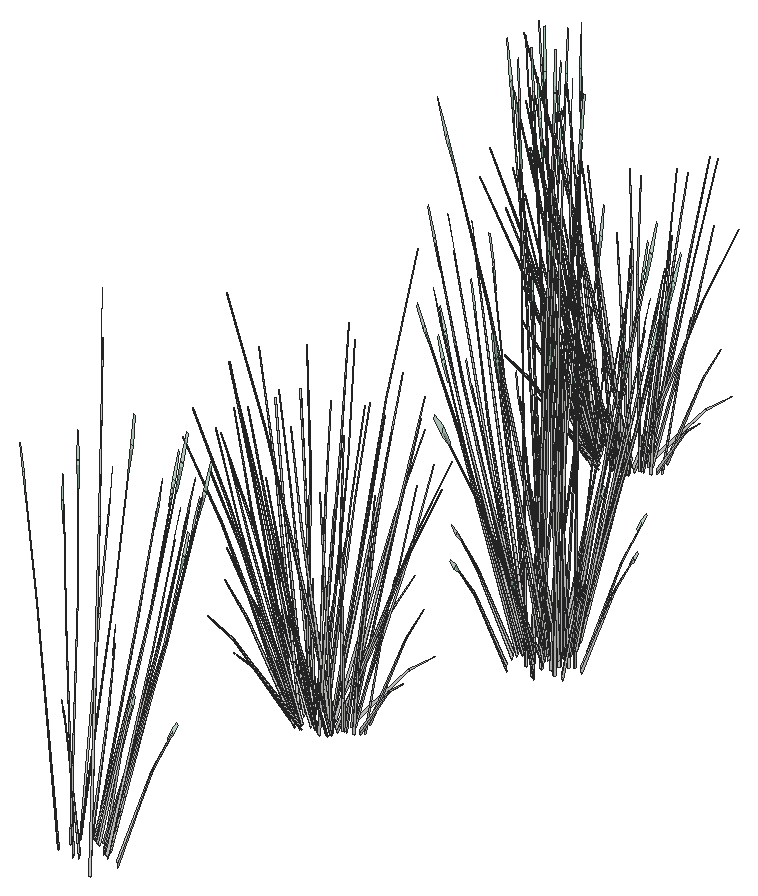
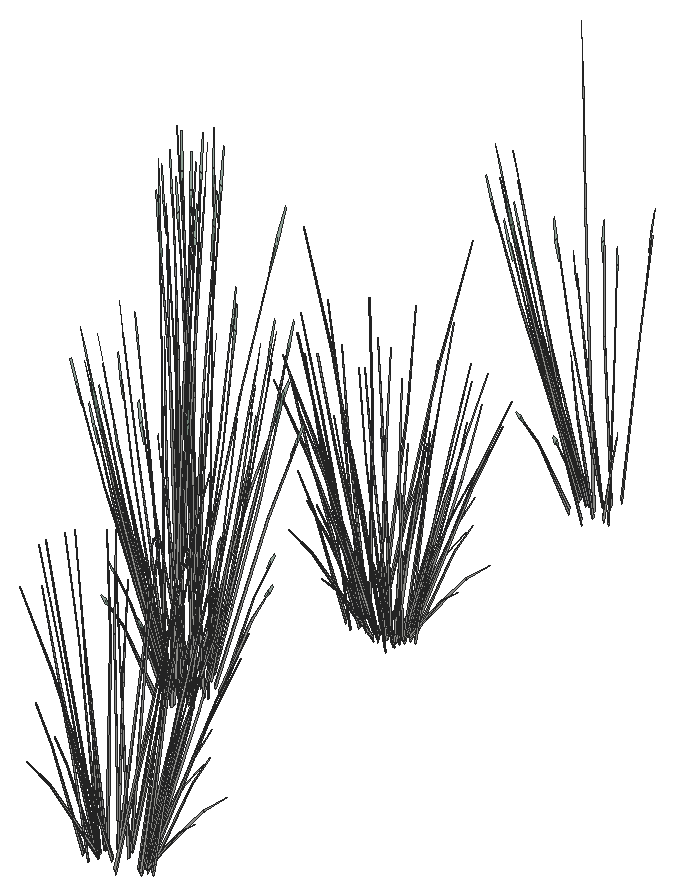
# SketchUp Ruby script. Lengths in inches.
U = 1.inch
M = Sketchup.active_model
def pt(a) = Geom::Point3d.new(a.map { |v| v * U })
def face(e, loops, mat)
  f = e.add_face(loops[0].map { |a| pt(a) })
  loops[1..].each { |l| e.add_face(l.map { |a| pt(a) }).erase! }
  f.material = f.back_material = mat if mat
  f
end
# faces: each face lists its corners as indices into pts; further lists are holes
def faces(e, pts, list, mat = nil) = list.each { |f| face(e, (f[0].is_a?(Array) ? f : [f]).map { |l| l.map { |i| pts[i] } }, mat) }
# xy, xz, yz: faces in a plane at the given z, y or x. An outline is a flat list of corners, or four numbers for a rectangle; further outlines are holes
def ring(l) = l.size == 4 ? [[l[0], l[1]], [l[2], l[1]], [l[2], l[3]], [l[0], l[3]]] : l.each_slice(2).to_a
def flat(e, list, mat, &to3) = list.each { |f| face(e, (f[0].is_a?(Array) ? f : [f]).map { |l| ring(l).map { |u, v| to3.(u, v) } }, mat) }
def xy(e, z, list, mat = nil) = flat(e, list, mat) { |x, y| [x, y, z] }
def xz(e, y, list, mat = nil) = flat(e, list, mat) { |x, z| [x, y, z] }
def yz(e, x, list, mat = nil) = flat(e, list, mat) { |y, z| [x, y, z] }
def lines(e, pts, list) = list.each { |a, b| e.add_line(pt(pts[a]), pt(pts[b])) }
# prism: a flat outline (further loops are holes) pulled along v
def prism(e, loops, v, mat = nil)
  f = face(e, loops, mat); d = Geom::Vector3d.new(v.map { |x| x * U })
  f.pushpull(f.normal.samedirection?(d) ? d.length : -d.length)
end
def box(e, o, s, mat = nil) = prism(e, [[o, [o[0] + s[0], o[1], o[2]], [o[0] + s[0], o[1] + s[1], o[2]], [o[0], o[1] + s[1], o[2]]]], [0, 0, s[2]], mat)
def at(x, y, z, deg = 0) = Geom::Transformation.translation(pt([x, y, z])) * Geom::Transformation.rotation(ORIGIN, Z_AXIS, deg.degrees)
def axes(o, x, y, z) = Geom::Transformation.new([*x, 0, *y, 0, *z, 0, *pt(o).to_a, 1])
def part(name) = M.definitions.add(name)
# library, detail: a bought-in or finely detailed component or shape, given as its bounding box
def library(name, o, s) = part(name).tap { |d| box(d.entities, o, s) }
def detail(e, o, s) = box(e.add_group.entities, o, s)
def put(e, d, t, mat = nil) = e.add_instance(d, t).tap { |i| i.material = mat if mat }
def group(e, t, mat = nil) = e.add_group.tap { |g| g.transformation = t; g.material = mat if mat }.entities
root = M.entities
M.materials.add("LightPink_Translucent").color = [175, 214, 192]
M.materials["LightPink_Translucent"].alpha = 0.75
c1 = part("blade")
p = [[2.15,0.21,22],[0,0.17,0],[0.09,0.45,0],[2.18,0.31,22],[2.29,0.31,22],[0.38,0.45,0],
  [2.48,0.24,33],[2.49,0.24,33],[2.48,0.22,33]]
faces(c1.entities,p,[[0,1,2,3],[4,5,2,3],[6,3,4,7],[8,0,3,6]])
c2 = part("seeds")
p = [[0.3,-0.1,1.38],[-0.01,-0.03,1.59],[-0.01,-0.03,0.03],[0.14,-0.07,-0.07],[0.29,-0.03,3],[0.15,0.01,3.11]]
faces(c2.entities,p,[[0,1,2,3],[1,0,4,5]],"LightPink_Translucent")
c3 = part("blade with seeds")
put(c3.entities,c1,at(0,0,0))
put(c3.entities,c2,axes([2.4,0.25,30.99],[1.5799,-0.05474,1.17369],[-0.12525,1.92788,0.29478],[-0.07173,-0.02425,1.56792]))
c4 = part("blade with seeds\#1")
put(c4.entities,c1,at(0,0,0))
put(root,c3,axes([491.25,325.37,141.43],[-0.11164,0.46982,-0.465],[-0.38276,-0.16104,-0.36018],[-0.1541,0.04308,0.88973]))
put(root,c3,axes([493.54,325.76,139.64],[0.37379,-0.28711,0.40713],[0.26322,0.43489,-0.19594],[-0.04625,0.09291,1.30716]))
put(root,c3,axes([494.51,326.625,141.43],[0.29922,-0.34214,-0.465],[0.26205,0.36143,-0.36018],[0.15203,0.05206,0.88973]))
put(root,c3,axes([494.375,326.73,141.7],[0.41193,0.01244,-0.64651],[-0.02767,0.52368,0.07802],[0.17451,0.05527,0.91455]))
put(root,c3,axes([494.62,326.95,141.29],[0.23447,0.32338,-0.32227],[-0.26773,0.30612,0.41605],[0.13603,0.04658,0.79608]))
put(root,c3,axes([491.61,327.02,139.6875],[0.12805,-0.2691,1.04523],[0.13011,0.34747,0.76796],[-0.11021,0.09372,0.23022]))
put(root,c3,axes([491.02,327.07,139.6],[0.01397,-0.30649,0.95605],[0.29664,0.2024,0.52785],[-0.10539,0.12108,0.74993]))
put(root,c3,axes([491.43,326.42,141.43],[0.10586,0.47162,-0.465],[-0.4009,0.0825,-0.36018],[-0.11489,0.12667,0.88973]))
put(root,c3,axes([493.82,327.33,141.43],[0.40663,-0.12278,-0.465],[0.07113,0.46497,-0.36018],[0.10922,0.13325,0.88973]))
put(root,c3,axes([491.72,328.15,140.75],[0.37435,-0.09148,-0.03177],[0.08606,0.43236,-0.14407],[-0.02373,0.09029,0.47519]))
put(root,c3,axes([494.63,327.91,139.6875],[-0.2267,-0.15919,1.04523],[0.30457,-0.13683,0.76796],[0.07632,0.13148,0.23022]))
put(root,c3,axes([493.78,327.68,141.29],[0.06364,0.41603,-0.32227],[-0.36383,0.10985,0.41605],[0.09772,0.11922,0.79608]))
put(root,c3,axes([493.66,327.35,141.7],[0.35138,0.24965,-0.64651],[-0.24972,0.43748,0.07802],[0.12731,0.14906,0.91455]))
put(root,c3,axes([491.77,327.34,141.29],[-0.27882,0.27194,-0.32227],[-0.26394,-0.31051,0.41605],[-0.04016,0.15777,0.79608]))
put(root,c3,axes([492.92,327.55,141.43],[0.40508,0.12948,-0.465],[-0.13885,0.44393,-0.36018],[0.03714,0.17873,0.88973]))
put(root,c3,axes([492.66,328.67,139.6875],[-0.07352,-0.2953,1.04523],[0.30384,0.139,0.76796],[-0.02079,0.15666,0.23022]))
put(root,c3,axes([492.73,327.82,141.29],[-0.12423,0.3972,-0.32227],[-0.36244,-0.11585,0.41605],[0.03323,0.15992,0.79608]))
put(root,c3,axes([491.95,327.06,141.7],[-0.01072,0.47777,-0.64651],[-0.45152,-0.03209,0.07802],[-0.04765,0.2024,0.91455]))
put(root,c3,axes([492.77,327.47,141.7],[0.19668,0.41997,-0.64651],[-0.40486,0.23405,0.07802],[0.04599,0.20292,0.91455]))
put(root,c4,axes([492.47,352.11,139.99],[0.11364,0.12234,1.40588],[-0.52511,0.103,0.11368],[-0.11868,-0.19206,0.601]))
put(root,c4,axes([493.34,351.3,140.68],[-0.07604,-0.05342,1.43516],[-0.50744,0.03387,-0.22697],[-0.08099,-0.12778,0.1151]))
put(root,c4,axes([495.51,351.68,140.68],[-0.05049,0.0291,1.45516],[-0.49465,-0.09819,-0.1375],[-0.01791,-0.12701,0.25751]))
put(root,c4,axes([495.62,351.95,140.68],[-0.0048,-0.07584,1.43516],[-0.40531,-0.21918,-0.22697],[0.06266,-0.13286,0.1151]))
put(root,c4,axes([494.25,352.32,139.99],[-0.09256,0.13097,1.40588],[-0.38832,-0.27104,0.11368],[0.17518,-0.16893,0.601]))
put(root,c4,axes([493.92,351.9375,140.53],[0.14987,-0.29303,-0.29052],[0.43725,0.08547,0.37506],[-0.04009,-0.11798,0.71765]))
put(root,c4,axes([492.82,351.12,140.68],[-0.00927,0.04567,1.45516],[-0.45742,0.16576,-0.1375],[-0.1346,-0.08473,0.25751]))
put(root,c4,axes([494.11,352.12,140.94],[-0.48648,0.17741,-0.09976],[-0.23906,-0.31487,-0.55369],[-0.06419,-0.13269,0.84132]))
put(root,c4,axes([495.12,352.52,140.94],[-0.54637,-0.01888,-0.09976],[0.01493,-0.35746,-0.55369],[0.03795,-0.13767,0.84132]))
put(root,c4,axes([492.66,352.04,140.53],[-0.07678,-0.30692,-0.29052],[0.43892,-0.08104,0.37506],[-0.11789,-0.08795,0.71765]))
put(root,c4,axes([495.08,352.29,140.53],[0.33637,-0.20062,-0.29052],[0.31842,0.22908,0.37506],[0.04845,-0.11639,0.71765]))
put(root,c4,axes([491.71,352.49,139.99],[0.18466,0.06565,1.40588],[-0.38215,0.27542,0.11368],[-0.23818,-0.12424,0.601]))
put(root,c4,axes([491.67,351.89,140.68],[-0.10696,-0.00269,1.43516],[-0.34054,0.26896,-0.22697],[-0.1817,-0.05496,0.1151]))
put(root,c4,axes([495.72,353.22,140.94],[-0.45986,-0.21011,-0.09976],[0.26493,-0.30427,-0.55369],[0.12992,-0.10577,0.84132]))
put(root,c4,axes([496.85,353.13,140.68],[-0.06493,-0.00289,1.45516],[-0.26964,-0.31009,-0.1375],[0.10828,-0.10196,0.25751]))
put(root,c4,axes([493.82,354.37,139.54],[0.4296,0.15365,1.24087],[-0.42086,0.33102,0.4907],[-0.18851,-0.19619,1.04025]))
put(root,c4,axes([491.64,352.58,140.53],[-0.28286,-0.23857,-0.29052],[0.32298,-0.22584,0.37506],[-0.1641,-0.03436,0.71765]))
put(root,c4,axes([495.84,353.01,140.53],[0.43273,-0.05446,-0.29052],[0.11427,0.31131,0.37506],[0.12401,-0.08362,0.71765]))
put(root,c4,axes([497.09,353.5,140.68],[0.06898,-0.05804,1.43516],[-0.0883,-0.35603,-0.22697],[0.17309,-0.0675,0.1151]))
put(root,c4,axes([491.26,352.11,140.68],[0.03685,0.03803,1.45516],[-0.17767,0.34183,-0.1375],[-0.17994,0.00247,0.25751]))
put(root,c4,axes([491.96,352.56,140.94],[-0.02662,0.38751,-0.09976],[-0.50399,-0.01059,-0.55369],[-0.19411,-0.02692,0.84132]))
put(root,c4,axes([495.73,354.04,140.94],[-0.25013,-0.34504,-0.09976],[0.44394,-0.16956,-0.55369],[0.18708,-0.04552,0.84132]))
put(root,c4,axes([491.32,353.09,139.99],[0.2062,-0.00863,1.40588],[-0.13679,0.37404,0.11368],[-0.29386,-0.02314,0.601]))
put(root,c4,axes([491.14,353.41,140.53],[-0.41315,-0.1063,-0.29052],[0.1205,-0.31012,0.37506],[-0.16634,0.02844,0.71765]))
put(root,c4,axes([496,353.91,140.53],[0.41315,0.1063,-0.29052],[-0.1205,0.31012,0.37506],[0.16634,-0.02844,0.71765]))
put(root,c4,axes([494.87,353.52,139.99],[-0.2062,0.00863,1.40588],[0.13679,-0.37404,0.11368],[0.29386,0.02314,0.601]))
put(root,c4,axes([492.4,353.36,139.55],[0.14131,-0.05512,1.45254],[0.04873,0.38487,0.11368],[-0.30608,0.05107,0.51915]))
put(root,c4,axes([491.4,353.27,140.94],[0.25013,0.34504,-0.09976],[-0.44394,0.16956,-0.55369],[-0.18708,0.04552,0.84132]))
put(root,c4,axes([496.73,355.07,140.68],[-0.04495,-0.03336,1.45516],[0.09833,-0.35758,-0.1375],[0.17707,-0.02285,0.25751]))
put(root,c4,axes([490.88,353.62,140.68],[-0.08118,0.04947,1.43516],[0.00691,0.36146,-0.22697],[-0.18608,0.04701,0.1151]))
put(root,c4,axes([496.34,354.77,140.04],[-0.09515,-0.32031,-0.02864],[0.44972,-0.07364,-0.12987],[0.09391,0.02031,0.42837]))
put(root,c4,axes([495.17,354.76,140.94],[0.02662,-0.38751,-0.09976],[0.50399,0.01059,-0.55369],[0.19411,0.02692,0.84132]))
put(root,c4,axes([495.61,354.53,140.68],[0.10664,-0.00644,1.43516],[0.29251,-0.29603,-0.22697],[0.18969,0.03908,0.1151]))
put(root,c4,axes([491.41,353.75,139.99],[0.17249,-0.0806,1.40588],[0.14522,0.37244,0.11368],[-0.2708,0.08417,0.601]))
put(root,c4,axes([489.98,353.98,140.68],[0.06344,0.01022,1.45516],[0.19627,0.33667,-0.1375],[-0.12987,0.08837,0.25751]))
put(root,c4,axes([491.29,354.31,140.53],[-0.43273,0.05446,-0.29052],[-0.11427,-0.31131,0.37506],[-0.12401,0.08362,0.71765]))
put(root,c4,axes([495.5,354.73,140.53],[0.28286,0.23857,-0.29052],[-0.32298,0.22584,0.37506],[0.1641,0.03436,0.71765]))
put(root,c4,axes([494.52,353.26,140.48],[-0.42958,-0.19798,1.1344],[0.45359,-0.30825,0.48946],[0.1386,0.18577,1.09651]))
put(root,c4,axes([494.48,354.12,139.99],[-0.18466,-0.06565,1.40588],[0.38215,-0.27542,0.11368],[0.23818,0.12424,0.601]))
put(root,c4,axes([491.42,354.09,140.94],[0.45986,0.21011,-0.09976],[-0.26493,0.30427,-0.55369],[-0.12992,0.10577,0.84132]))
put(root,c4,axes([492.04,354,139.99],[0.12417,-0.11708,1.40588],[0.31352,0.31602,0.11368],[-0.21504,0.14392,0.601]))
put(root,c4,axes([494.18,355.18,140.94],[0.29624,-0.32616,-0.09976],[0.42901,0.1879,-0.55369],[0.14913,0.09215,0.84132]))
put(root,c4,axes([493.79,355.45,140.68],[0.00147,-0.04613,1.45516],[0.42603,-0.20353,-0.1375],[0.14798,0.07265,0.25751]))
put(root,c4,axes([491.94,354.29,139.99],[0.09256,-0.13097,1.40588],[0.38832,0.27104,0.11368],[-0.17518,0.16893,0.601]))
put(root,c4,axes([492.05,355.03,140.53],[-0.33637,0.20062,-0.29052],[-0.31842,-0.22908,0.37506],[-0.04845,0.11639,0.71765]))
put(root,c4,axes([490.89,354.97,140.68],[-0.01236,0.0754,1.43516],[0.35069,0.26232,-0.22697],[-0.09181,0.12405,0.1151]))
put(root,c4,axes([493.02,355.2,140.94],[0.48648,-0.17741,-0.09976],[0.23906,0.31487,-0.55369],[0.06419,0.13269,0.84132]))
put(root,c4,axes([492.39,354.93,140.92],[0.35588,0.25603,-0.4653],[-0.37594,0.22422,-0.36041],[-0.05415,0.13008,0.89031]))
put(root,c4,axes([493.72,354.5,139.99],[-0.11364,-0.12234,1.40588],[0.52511,-0.103,0.11368],[0.11868,0.19206,0.601]))
put(root,c4,axes([493.22,355.38,140.53],[-0.14987,0.29303,-0.29052],[-0.43725,-0.08547,0.37506],[0.04009,0.11798,0.71765]))
put(root,c4,axes([492.28,354.82,141.19],[-0.01294,0.35246,-0.64693],[-0.54471,-0.02367,0.07807],[-0.05748,0.14932,0.91515]))
put(root,c4,axes([492.79,354.57,139.99],[-0.01217,-0.14625,1.40588],[0.52737,0.09702,0.11368],[-0.03262,0.20842,0.601]))
put(root,c4,axes([490.85,355.74,140.68],[0.0564,-0.02301,1.45516],[0.46615,0.15302,-0.1375],[-0.01095,0.12741,0.25751]))
put(root,c4,axes([492.91,355.9,140.68],[0.06302,0.06136,1.43516],[0.50855,0.02411,-0.22697],[0.05114,0.13532,0.1151]))
put(root,c4,axes([492.09,355.3125,139.57],[0.01092,-0.19671,1.26617],[0.49126,0.1039,0.17497],[-0.04257,0.20964,0.59789]))
put(root,c3,axes([500.8125,370.27,140.31],[0.06442,0.13585,1.61128],[-0.4498,0.04685,0.1261],[-0.05969,-0.29426,0.57588]))
put(root,c3,axes([501.54,369.83,141.8],[0.01072,-0.47777,-0.64651],[0.45152,0.03209,0.07802],[0.04765,-0.2024,0.91455]))
put(root,c3,axes([500.75,369.0625,141.38],[0.12423,-0.3972,-0.32227],[0.36244,0.11585,0.41605],[-0.03323,-0.15992,0.79608]))
put(root,c3,axes([500.57,369.33,141.52],[-0.40508,-0.12948,-0.465],[0.13885,-0.44393,-0.36018],[-0.03714,-0.17873,0.88973]))
put(root,c3,axes([501.44,369.67,141.52],[-0.29499,-0.34704,-0.465],[0.31162,-0.30393,-0.36018],[0.04488,-0.17633,0.88973]))
put(root,c3,axes([498.84,368.45,139.78],[0.20183,0.19918,1.04523],[-0.31952,0.0786,0.76796],[-0.05721,-0.14394,0.23022]))
put(root,c3,axes([501.72,369.54,141.38],[0.27882,-0.27194,-0.32227],[0.26394,0.31051,0.41605],[0.04016,-0.15777,0.79608]))
put(root,c3,axes([499.71,369.21,141.38],[-0.06364,-0.41603,-0.32227],[0.36383,-0.10985,0.41605],[-0.09772,-0.11922,0.79608]))
put(root,c3,axes([501.05,368.89,139.78],[0.03187,0.30513,1.04523],[-0.28077,-0.19355,0.76796],[0.04212,-0.15079,0.23022]))
put(root,c3,axes([499.67,369.55,141.52],[-0.40663,0.12278,-0.465],[-0.07113,-0.46497,-0.36018],[-0.10922,-0.13325,0.88973]))
put(root,c3,axes([502.07,370.66,141.8],[0.21525,-0.40754,-0.64651],[0.37719,0.28963,0.07802],[0.12852,-0.14765,0.91455]))
put(root,c3,axes([502.06,370.47,141.52],[-0.10586,-0.47162,-0.465],[0.4009,-0.0825,-0.36018],[0.11489,-0.12667,0.88973]))
put(root,c3,axes([502.35,370.52,141.38],[0.3587,-0.07382,-0.32227],[0.09472,0.42197,0.41605],[0.10279,-0.11334,0.79608]))
put(root,c3,axes([498.87,369.9375,141.38],[-0.23447,-0.32338,-0.32227],[0.26773,-0.30612,0.41605],[-0.13603,-0.04658,0.79608]))
put(root,c3,axes([499.63,371.63,140.29],[-0.17958,0.41302,1.37647],[-0.38687,-0.40462,0.54432],[0.22929,-0.18124,1.15394]))
put(root,c3,axes([502.89,370.06,139.78],[-0.155,0.24931,1.04523],[-0.09317,-0.36309,0.76796],[0.11912,-0.07769,0.23022]))
put(root,c3,axes([499.11,370.15,142.125],[-0.41193,-0.01244,-0.71763],[0.02767,-0.52368,0.0866],[-0.17451,-0.05527,1.01516]))
put(root,c3,axes([497.96,370.14,139.78],[0.2648,-0.01237,1.04523],[-0.18886,0.30908,0.76796],[-0.12621,-0.06079,0.23022]))
put(root,c3,axes([499.07,370.59,139.52],[-0.22267,0.44731,0.45182],[-0.39927,-0.26736,0],[0.05071,-0.10188,1.43328]))
put(root,c3,axes([498.53,369.98,140.33],[0.22989,0.0105,1.40454],[-0.12143,0.4723,0.19409],[-0.24501,-0.04092,0.66323]))
put(root,c3,axes([500.46,369.7,139.52],[-0.44533,0,0.45182],[0,-0.53472,0],[0.10143,0,1.43328]))
put(root,c3,axes([498.98,370.26,141.82],[-0.29922,0.34214,-0.51615],[-0.26205,-0.36143,-0.3998],[-0.15203,-0.05206,0.9876]))
put(root,c3,axes([500.49,372.27,139.85],[0.4193,-0.01306,1.28558],[-0.10869,0.59089,0.54432],[-0.22943,-0.13975,1.21348]))
put(root,c3,axes([502.24,371.52,141.52],[0.11164,-0.46982,-0.465],[0.38276,0.16104,-0.36018],[0.1541,-0.04308,0.88973]))
put(root,c3,axes([500.24,370.92,139.74],[-0.40128,-0.23189,0.40713],[0.19312,-0.48183,-0.19594],[0.0925,0,1.30716]))
put(root,c3,axes([502.17,371.6875,141.8],[0.3621,-0.22811,-0.64651],[0.2018,0.46957,0.07802],[0.17496,-0.05334,0.91455]))
put(root,c3,axes([499.29,370.75,139.52],[0.1182,0.51358,0.16054],[-0.43988,0.12682,0.31929],[0.06409,-0.0458,1.4597]))
put(root,c3,axes([499.27,372.28,139.52],[0.44258,0.13807,0.16054],[-0.12525,0.50524,0.31929],[-0.00216,-0.08728,1.4597]))
put(root,c3,axes([500.05,372.04,139.74],[0.02749,0.519,0.40713],[-0.45634,0.04694,-0.19594],[-0.04625,-0.09291,1.30716]))
put(root,c3,axes([499.03,372.42,139.52],[0.22267,0.44731,0.45182],[-0.39927,0.26736,0],[-0.05071,-0.10188,1.43328]))
put(root,c3,axes([502.48,371.73,141.38],[0.34247,0.14409,-0.32227],[-0.09989,0.42037,0.41605],[0.13788,-0.03855,0.79608]))
put(root,c3,axes([498.45,371.06,141.38],[-0.34247,-0.14409,-0.32227],[0.09989,-0.42037,0.41605],[-0.13788,0.03855,0.79608]))
put(root,c3,axes([500.4,373.07,139.52],[0.32439,-0.37551,0.16054],[0.31463,0.37842,0.31929],[-0.06625,-0.04147,1.4597]))
put(root,c3,axes([500.79,371.04,139.74],[-0.02749,-0.519,0.40713],[0.45634,-0.04694,-0.19594],[0.04625,0.09291,1.30716]))
put(root,c3,axes([501.58,370.8,139.52],[-0.44258,-0.13807,0.16054],[0.12525,-0.50524,0.31929],[0.00216,0.08728,1.4597]))
put(root,c3,axes([498.76,371.1,141.8],[-0.3621,0.22811,-0.64651],[-0.2018,-0.46957,0.07802],[-0.17496,0.05334,0.91455]))
put(root,c3,axes([501.55,372.33,139.52],[-0.1182,-0.51358,0.16054],[0.43988,-0.12682,0.31929],[-0.06409,0.0458,1.4597]))
put(root,c3,axes([503.2,371.81,139.78],[-0.25968,0.06131,1.04523],[0.14383,-0.34012,0.76796],[0.13297,0.0366,0.23022]))
put(root,c3,axes([500.61,372.16,139.74],[0.40128,0.23189,0.40713],[-0.19312,0.48183,-0.19594],[-0.0925,0,1.30716]))
put(root,c3,axes([498.6875,371.27,141.52],[-0.11164,0.46982,-0.465],[-0.38276,-0.16104,-0.36018],[-0.1541,0.04308,0.88973]))
put(root,c3,axes([500.98,371.66,139.74],[0.37379,-0.28711,0.40713],[0.26322,0.43489,-0.19594],[-0.04625,0.09291,1.30716]))
put(root,c3,axes([501.95,372.53,141.52],[0.29922,-0.34214,-0.465],[0.26205,0.36143,-0.36018],[0.15203,0.05206,0.88973]))
put(root,c3,axes([500.39,373.38,139.52],[0.44533,0,0.45182],[0,0.53472,0],[-0.10143,0,1.43328]))
put(root,c3,axes([501.78,372.5,139.52],[0.22267,-0.44731,0.45182],[0.39927,0.26736,0],[-0.05071,0.10188,1.43328]))
put(root,c3,axes([501.82,372.64,141.8],[0.41193,0.01244,-0.64651],[-0.02767,0.52368,0.07802],[0.17451,0.05527,0.91455]))
put(root,c3,axes([502.0625,372.85,141.38],[0.23447,0.32338,-0.32227],[-0.26773,0.30612,0.41605],[0.13603,0.04658,0.79608]))
put(root,c3,axes([499.05,372.93,139.78],[0.12805,-0.2691,1.04523],[0.13011,0.34747,0.76796],[-0.11021,0.09372,0.23022]))
put(root,c3,axes([498.47,372.97,139.69],[0.01397,-0.30649,0.95605],[0.29664,0.2024,0.52785],[-0.10539,0.12108,0.74993]))
put(root,c3,axes([498.875,372.32,141.52],[0.10586,0.47162,-0.465],[-0.4009,0.0825,-0.36018],[-0.11489,0.12667,0.88973]))
put(root,c3,axes([501.26,373.24,141.52],[0.40663,-0.12278,-0.465],[0.07113,0.46497,-0.36018],[0.10922,0.13325,0.88973]))
put(root,c3,axes([502.07,373.8125,139.78],[-0.2267,-0.15919,1.04523],[0.30457,-0.13683,0.76796],[0.07632,0.13148,0.23022]))
put(root,c3,axes([501.22,373.58,141.38],[0.06364,0.41603,-0.32227],[-0.36383,0.10985,0.41605],[0.09772,0.11922,0.79608]))
put(root,c3,axes([501.1,373.25,141.8],[0.35138,0.24965,-0.64651],[-0.24972,0.43748,0.07802],[0.12731,0.14906,0.91455]))
put(root,c3,axes([499.21,373.25,141.38],[-0.27882,0.27194,-0.32227],[-0.26394,-0.31051,0.41605],[-0.04016,0.15777,0.79608]))
put(root,c3,axes([500.36,373.46,141.52],[0.40508,0.12948,-0.465],[-0.13885,0.44393,-0.36018],[0.03714,0.17873,0.88973]))
put(root,c3,axes([500.1,374.57,139.78],[-0.07352,-0.2953,1.04523],[0.30384,0.139,0.76796],[-0.02079,0.15666,0.23022]))
put(root,c3,axes([500.18,373.73,141.38],[-0.12423,0.3972,-0.32227],[-0.36244,-0.11585,0.41605],[0.03323,0.15992,0.79608]))
put(root,c3,axes([499.4,372.96,141.8],[-0.01072,0.47777,-0.64651],[-0.45152,-0.03209,0.07802],[-0.04765,0.2024,0.91455]))
put(root,c3,axes([500.21,373.37,141.8],[0.19668,0.41997,-0.64651],[-0.40486,0.23405,0.07802],[0.04599,0.20292,0.91455]))
put(root,c4,axes([485.03,396.32,139.9],[0.11364,0.12234,1.40588],[-0.52511,0.103,0.11368],[-0.11868,-0.19206,0.601]))
put(root,c4,axes([485.9,395.51,140.59],[-0.07604,-0.05342,1.43516],[-0.50744,0.03387,-0.22697],[-0.08099,-0.12778,0.1151]))
put(root,c4,axes([488.07,395.89,140.58],[-0.05049,0.0291,1.45516],[-0.49465,-0.09819,-0.1375],[-0.01791,-0.12701,0.25751]))
put(root,c4,axes([488.18,396.17,140.59],[-0.0048,-0.07584,1.43516],[-0.40531,-0.21918,-0.22697],[0.06266,-0.13286,0.1151]))
put(root,c4,axes([486.8,396.54,139.9],[-0.09256,0.13097,1.40588],[-0.38832,-0.27104,0.11368],[0.17518,-0.16893,0.601]))
put(root,c4,axes([486.47,396.15,140.43],[0.14987,-0.29303,-0.29052],[0.43725,0.08547,0.37506],[-0.04009,-0.11798,0.71765]))
put(root,c4,axes([485.375,395.34,140.58],[-0.00927,0.04567,1.45516],[-0.45742,0.16576,-0.1375],[-0.1346,-0.08473,0.25751]))
put(root,c4,axes([486.67,396.34,140.85],[-0.48648,0.17741,-0.09976],[-0.23906,-0.31487,-0.55369],[-0.06419,-0.13269,0.84132]))
put(root,c4,axes([486.53,396.22,140.6],[0.48986,0.09962,0.39379],[-0.16751,0.3275,0.3247],[-0.02944,-0.12879,0.81485]))
put(root,c4,axes([487.68,396.73,140.85],[-0.54637,-0.01888,-0.09976],[0.01493,-0.35746,-0.55369],[0.03795,-0.13767,0.84132]))
put(root,c4,axes([485.21,396.26,140.43],[-0.07678,-0.30692,-0.29052],[0.43892,-0.08104,0.37506],[-0.11789,-0.08795,0.71765]))
put(root,c4,axes([487.64,396.5,140.43],[0.33637,-0.20062,-0.29052],[0.31842,0.22908,0.37506],[0.04845,-0.11639,0.71765]))
put(root,c4,axes([484.27,396.7,139.9],[0.18466,0.06565,1.40588],[-0.38215,0.27542,0.11368],[-0.23818,-0.12424,0.601]))
put(root,c4,axes([485.5,396.2,141.17],[-0.33178,0.3653,-0.11173],[-0.48049,-0.21045,-0.62013],[-0.16702,-0.10321,0.94228]))
put(root,c4,axes([487.64,396.58,140.6],[0.354,0.25999,0.39379],[-0.37594,0.22422,0.3247],[0.0653,-0.12198,0.81485]))
put(root,c4,axes([484.23,396.1,140.59],[-0.10696,-0.00269,1.43516],[-0.34054,0.26896,-0.22697],[-0.1817,-0.05496,0.1151]))
put(root,c4,axes([488.27,397.4375,140.85],[-0.45986,-0.21011,-0.09976],[0.26493,-0.30427,-0.55369],[0.12992,-0.10577,0.84132]))
put(root,c4,axes([489.41,397.35,140.58],[-0.06493,-0.00289,1.45516],[-0.26964,-0.31009,-0.1375],[0.10828,-0.10196,0.25751]))
put(root,c4,axes([486.375,398.58,139.45],[0.4296,0.15365,1.24087],[-0.42086,0.33102,0.4907],[-0.18851,-0.19619,1.04025]))
put(root,c4,axes([484.2,396.8,140.43],[-0.28286,-0.23857,-0.29052],[0.32298,-0.22584,0.37506],[-0.1641,-0.03436,0.71765]))
put(root,c4,axes([488.4,397.23,140.43],[0.43273,-0.05446,-0.29052],[0.11427,0.31131,0.37506],[0.12401,-0.08362,0.71765]))
put(root,c4,axes([488.35,397.29,140.6],[0.12329,0.35069,0.39379],[-0.48364,0.06086,0.3247],[0.14254,-0.08248,0.81485]))
put(root,c4,axes([489.65,397.72,140.59],[0.06898,-0.05804,1.43516],[-0.0883,-0.35603,-0.22697],[0.17309,-0.0675,0.1151]))
put(root,c4,axes([483.82,396.33,140.58],[0.03685,0.03803,1.45516],[-0.17767,0.34183,-0.1375],[-0.17994,0.00247,0.25751]))
put(root,c4,axes([484.52,396.77,140.85],[-0.02662,0.38751,-0.09976],[-0.50399,-0.01059,-0.55369],[-0.19411,-0.02692,0.84132]))
put(root,c4,axes([488.29,398.26,140.85],[-0.25013,-0.34504,-0.09976],[0.44394,-0.16956,-0.55369],[0.18708,-0.04552,0.84132]))
put(root,c4,axes([483.88,397.3,139.9],[0.2062,-0.00863,1.40588],[-0.13679,0.37404,0.11368],[-0.29386,-0.02314,0.601]))
put(root,c4,axes([483.79,397.59,140.6],[0.14045,-0.34743,0.39379],[0.46175,0.1188,0.3247],[-0.18159,0.02088,0.81485]))
put(root,c4,axes([483.7,397.625,140.43],[-0.41315,-0.1063,-0.29052],[0.1205,-0.31012,0.37506],[-0.16634,0.02844,0.71765]))
put(root,c4,axes([488.55,398.12,140.43],[0.41315,0.1063,-0.29052],[-0.1205,0.31012,0.37506],[0.16634,-0.02844,0.71765]))
put(root,c4,axes([487.43,397.74,139.9],[-0.2062,0.00863,1.40588],[0.13679,-0.37404,0.11368],[0.29386,0.02314,0.601]))
put(root,c4,axes([488.46,398.16,140.6],[-0.14045,0.34743,0.39379],[-0.46175,-0.1188,0.3247],[0.18159,-0.02088,0.81485]))
put(root,c4,axes([483.96,397.49,140.85],[0.25013,0.34504,-0.09976],[-0.44394,0.16956,-0.55369],[-0.18708,0.04552,0.84132]))
put(root,c4,axes([489.29,399.28,140.58],[-0.04495,-0.03336,1.45516],[0.09833,-0.35758,-0.1375],[0.17707,-0.02285,0.25751]))
put(root,c4,axes([483.4375,397.83,140.59],[-0.08118,0.04947,1.43516],[0.00691,0.36146,-0.22697],[-0.18608,0.04701,0.1151]))
put(root,c4,axes([488.9,398.98,139.94],[-0.09515,-0.32031,-0.02864],[0.44972,-0.07364,-0.12987],[0.09391,0.02031,0.42837]))
put(root,c4,axes([487.73,398.97,140.85],[0.02662,-0.38751,-0.09976],[0.50399,0.01059,-0.55369],[0.19411,0.02692,0.84132]))
put(root,c4,axes([488.17,398.74,140.59],[0.10664,-0.00644,1.43516],[0.29251,-0.29603,-0.22697],[0.18969,0.03908,0.1151]))
put(root,c4,axes([483.9,398.45,140.6],[-0.12329,-0.35069,0.39379],[0.48364,-0.06086,0.3247],[-0.14254,0.08248,0.81485]))
put(root,c4,axes([483.96,397.96,139.9],[0.17249,-0.0806,1.40588],[0.14522,0.37244,0.11368],[-0.2708,0.08417,0.601]))
put(root,c4,axes([482.53,398.2,140.58],[0.06344,0.01022,1.45516],[0.19627,0.33667,-0.1375],[-0.12987,0.08837,0.25751]))
put(root,c4,axes([483.85,398.52,140.43],[-0.43273,0.05446,-0.29052],[-0.11427,-0.31131,0.37506],[-0.12401,0.08362,0.71765]))
